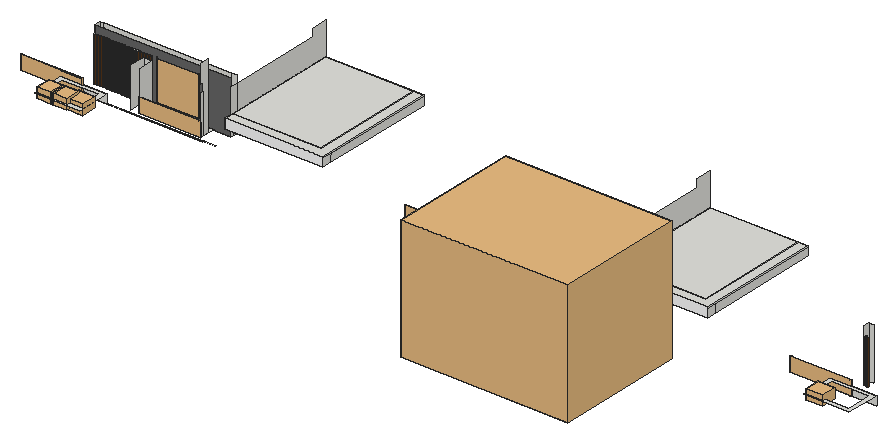
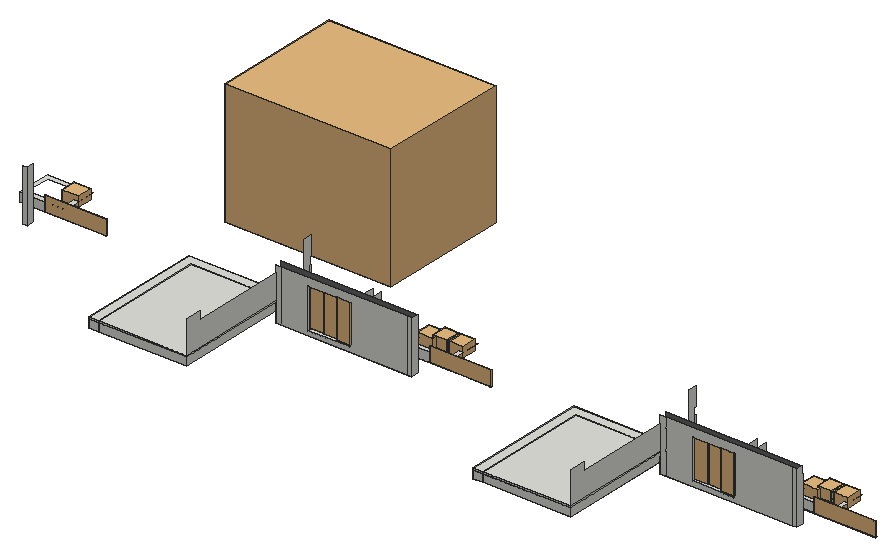
# SketchUp Ruby script. Lengths in inches.
U = 1.inch
M = Sketchup.active_model
def pt(a) = Geom::Point3d.new(a.map { |v| v * U })
def face(e, loops, mat)
  f = e.add_face(loops[0].map { |a| pt(a) })
  loops[1..].each { |l| e.add_face(l.map { |a| pt(a) }).erase! }
  f.material = f.back_material = mat if mat
  f
end
# faces: each face lists its corners as indices into pts; further lists are holes
def faces(e, pts, list, mat = nil) = list.each { |f| face(e, (f[0].is_a?(Array) ? f : [f]).map { |l| l.map { |i| pts[i] } }, mat) }
# xy, xz, yz: faces in a plane at the given z, y or x. An outline is a flat list of corners, or four numbers for a rectangle; further outlines are holes
def ring(l) = l.size == 4 ? [[l[0], l[1]], [l[2], l[1]], [l[2], l[3]], [l[0], l[3]]] : l.each_slice(2).to_a
def flat(e, list, mat, &to3) = list.each { |f| face(e, (f[0].is_a?(Array) ? f : [f]).map { |l| ring(l).map { |u, v| to3.(u, v) } }, mat) }
def xy(e, z, list, mat = nil) = flat(e, list, mat) { |x, y| [x, y, z] }
def xz(e, y, list, mat = nil) = flat(e, list, mat) { |x, z| [x, y, z] }
def yz(e, x, list, mat = nil) = flat(e, list, mat) { |y, z| [x, y, z] }
def lines(e, pts, list) = list.each { |a, b| e.add_line(pt(pts[a]), pt(pts[b])) }
# prism: a flat outline (further loops are holes) pulled along v
def prism(e, loops, v, mat = nil)
  f = face(e, loops, mat); d = Geom::Vector3d.new(v.map { |x| x * U })
  f.pushpull(f.normal.samedirection?(d) ? d.length : -d.length)
end
def box(e, o, s, mat = nil) = prism(e, [[o, [o[0] + s[0], o[1], o[2]], [o[0] + s[0], o[1] + s[1], o[2]], [o[0], o[1] + s[1], o[2]]]], [0, 0, s[2]], mat)
def at(x, y, z, deg = 0) = Geom::Transformation.translation(pt([x, y, z])) * Geom::Transformation.rotation(ORIGIN, Z_AXIS, deg.degrees)
def axes(o, x, y, z) = Geom::Transformation.new([*x, 0, *y, 0, *z, 0, *pt(o).to_a, 1])
def part(name) = M.definitions.add(name)
# library, detail: a bought-in or finely detailed component or shape, given as its bounding box
def library(name, o, s) = part(name).tap { |d| box(d.entities, o, s) }
def detail(e, o, s) = box(e.add_group.entities, o, s)
def put(e, d, t, mat = nil) = e.add_instance(d, t).tap { |i| i.material = mat if mat }
def group(e, t, mat = nil) = e.add_group.tap { |g| g.transformation = t; g.material = mat if mat }.entities
root = M.entities
M.materials.add("Material~3").color = [123, 113, 102]
M.materials.add("[0030_OldLace]").color = [86, 53, 24]
M.materials.add("[0128_White]").color = [255, 255, 255]
M.materials.add("[Slate Light Tile]").color = [104, 104, 104]
M.materials.add("[Wood Veneer 01]").color = [120, 70, 37]
c1 = part("glass-railing")
detail(c1.entities,[0,0,0],[1.26,75.59,33.1875])
c2 = library("Ornamental+Grasses",[-8.33,-8.78,0],[17.11,15.88,10.63])
c3 = library("3DGeom~4_Defintion",[362.52,-15.59,12.6],[288.85,70.11,1000])
c4 = library("3 door",[0,0,0],[74.8,3.9375,43.31])
c5 = library("Sans+titre+(1)+(1)+(2)",[-30.91,-35.46,0],[63.51,67.02,85.79])
xy(root,162.75,[[411.09,845.35,827.91,846.1],[1291.04,845.35,1707.86,846.1],[636.22,888.83,636.22,890.39,634.63,890.39,634.63,888.95,629.22,888.95,629.22,890.39,627.63,890.39,627.63,888.95,622.22,888.95,622.22,890.39,620.63,890.39,620.63,888.95,615.22,888.95,615.22,890.39,613.63,890.39,613.63,888.95,608.22,888.95,608.22,890.39,606.63,890.39,606.63,888.95,601.22,888.95,601.22,890.39,599.63,890.39,599.63,888.95,594.22,888.95,594.22,890.39,592.63,890.39,592.63,888.95,587.22,888.95,587.22,890.39,585.63,890.39,585.63,888.95,580.22,888.95,580.22,890.39,578.63,890.39,578.63,888.95,573.22,888.95,573.22,890.39,571.63,890.39,571.63,888.95,566.22,888.95,566.22,890.39,564.63,890.39,564.63,888.95,559.22,888.95,559.22,890.39,557.63,890.39,557.63,888.95,552.22,888.95,552.22,890.39,550.57,890.39,550.57,888.95,545.16,888.95,545.16,905.7,857.125,905.7,857.125,890.39,676.63,890.39,676.63,888.83,671.22,888.83,671.22,890.39,669.63,890.39,669.63,888.83,664.22,888.83,664.22,890.39,662.63,890.39,662.63,888.83,657.22,888.83,657.22,890.39,655.63,890.39,655.63,888.83,650.22,888.83,650.22,890.39,648.63,890.39,648.63,888.83,643.22,888.83,643.22,890.39,641.63,890.39,641.63,888.83],[1516.16,888.83,1516.16,890.39,1514.58,890.39,1514.58,888.95,1509.16,888.95,1509.16,890.39,1507.58,890.39,1507.58,888.95,1502.16,888.95,1502.16,890.39,1500.58,890.39,1500.58,888.95,1495.16,888.95,1495.16,890.39,1493.58,890.39,1493.58,888.95,1488.16,888.95,1488.16,890.39,1486.58,890.39,1486.58,888.95,1481.16,888.95,1481.16,890.39,1479.58,890.39,1479.58,888.95,1474.16,888.95,1474.16,890.39,1472.58,890.39,1472.58,888.95,1467.16,888.95,1467.16,890.39,1465.58,890.39,1465.58,888.95,1460.16,888.95,1460.16,890.39,1458.58,890.39,1458.58,888.95,1453.16,888.95,1453.16,890.39,1451.58,890.39,1451.58,888.95,1446.16,888.95,1446.16,890.39,1444.58,890.39,1444.58,888.95,1439.16,888.95,1439.16,890.39,1437.58,890.39,1437.58,888.95,1432.16,888.95,1432.16,890.39,1430.52,890.39,1430.52,888.95,1425.1,888.95,1425.1,905.7,1737.07,905.7,1737.07,890.39,1556.58,890.39,1556.58,888.83,1551.16,888.83,1551.16,890.39,1549.58,890.39,1549.58,888.83,1544.16,888.83,1544.16,890.39,1542.58,890.39,1542.58,888.83,1537.16,888.83,1537.16,890.39,1535.58,890.39,1535.58,888.83,1530.16,888.83,1530.16,890.39,1528.58,890.39,1528.58,888.83,1523.16,888.83,1523.16,890.39,1521.58,890.39,1521.58,888.83]])
xy(root,163,[[827.91,845.35,857.125,846.1],[1707.86,845.35,1737.07,846.1]])
xy(root,173.4375,[[687.49,840.97,827.91,877.14],[1567.4375,840.97,1707.86,877.14],[687.6875,890.39,782.75,905.7],[1567.63,890.39,1662.7,905.7]])
xy(root,183.3125,[[[505.35,767.72,609.54,845.35],[514,776.37,600.89,836.7]],[[1385.29,767.72,1489.48,845.35],[1393.94,776.37,1480.84,836.7]],[[2265.24,767.72,2369.43,845.35],[2273.89,776.37,2360.78,836.7]]])
xy(root,186.75,[[1044.04,893.65,1050.1875,895.71],[1052.35,893.65,1058.5,895.71],[1923.98,893.65,1930.13,895.71],[1932.29,893.65,1938.44,895.71],[861.16,894.34,867.3125,895.71],
  [869.48,894.34,875.625,895.71],[877.79,894.34,883.9375,895.71],[886.1,894.34,892.25,895.71],[894.41,894.34,900.5625,895.71],[902.73,894.34,908.875,895.71],
  [911.04,894.34,917.1875,895.71],[919.35,894.34,925.5,895.71],[927.66,894.34,933.8125,895.71],[935.98,894.34,942.125,895.71],[944.29,894.34,950.4375,895.71],
  [952.6,894.34,958.75,895.71],[960.91,894.34,967.0625,895.71],[969.23,894.34,975.375,895.71],[977.54,894.34,983.6875,895.71],[985.85,894.34,992,895.71],
  [994.16,894.34,1000.3125,895.71],[1002.48,894.34,1008.625,895.71],[1010.79,894.34,1016.9375,895.71],[1019.1,894.34,1025.25,895.71],[1027.41,894.34,1033.5625,895.71],
  [1035.73,894.34,1041.875,895.71],[1741.11,894.34,1747.26,895.71],[1749.42,894.34,1755.57,895.71],[1757.73,894.34,1763.88,895.71],[1766.04,894.34,1772.19,895.71],
  [1774.36,894.34,1780.51,895.71],[1782.67,894.34,1788.82,895.71],[1790.98,894.34,1797.13,895.71],[1799.29,894.34,1805.44,895.71],[1807.61,894.34,1813.76,895.71],
  [1815.92,894.34,1822.07,895.71],[1824.23,894.34,1830.38,895.71],[1832.54,894.34,1838.69,895.71],[1840.86,894.34,1847.01,895.71],[1849.17,894.34,1855.32,895.71],
  [1857.48,894.34,1863.63,895.71],[1865.79,894.34,1871.94,895.71],[1874.11,894.34,1880.26,895.71],[1882.42,894.34,1888.57,895.71],[1890.73,894.34,1896.88,895.71],
  [1899.04,894.34,1905.19,895.71],[1907.36,894.34,1913.51,895.71],[1915.67,894.34,1921.82,895.71],[[857.125,895.71,1058.5,1160.85],[865.59,904.18,1047.28,1152.375]],[[1737.07,895.71,1938.44,1160.85],[1745.54,904.18,1927.22,1152.375]]])
xy(root,186.75,[[857.125,873.28,857.125,895.71,861.16,895.71,861.16,894.34,867.3125,894.34,867.3125,895.71,869.48,895.71,869.48,894.34,875.625,894.34,875.625,895.71,877.79,895.71,877.79,894.34,883.9375,894.34,883.9375,895.71,886.1,895.71,886.1,894.34,892.25,894.34,892.25,895.71,894.41,895.71,894.41,894.34,900.5625,894.34,900.5625,895.71,902.73,895.71,902.73,894.34,908.875,894.34,908.875,895.71,911.04,895.71,911.04,894.34,917.1875,894.34,917.1875,895.71,919.35,895.71,919.35,894.34,925.5,894.34,925.5,895.71,927.66,895.71,927.66,894.34,933.8125,894.34,933.8125,895.71,935.98,895.71,935.98,894.34,942.125,894.34,942.125,895.71,944.29,895.71,944.29,894.34,950.4375,894.34,950.4375,895.71,952.6,895.71,952.6,894.34,958.75,894.34,958.75,895.71,960.91,895.71,960.91,894.34,967.0625,894.34,967.0625,895.71,969.23,895.71,969.23,894.34,975.375,894.34,975.375,895.71,977.54,895.71,977.54,894.34,983.6875,894.34,983.6875,895.71,985.85,895.71,985.85,894.34,992,894.34,992,895.71,994.16,895.71,994.16,894.34,1000.3125,894.34,1000.3125,895.71,1002.48,895.71,1002.48,894.34,1008.625,894.34,1008.625,895.71,1010.79,895.71,1010.79,894.34,1016.9375,894.34,1016.9375,895.71,1019.1,895.71,1019.1,894.34,1025.25,894.34,1025.25,895.71,1027.41,895.71,1027.41,894.34,1033.5625,894.34,1033.5625,895.71,1035.73,895.71,1035.73,894.34,1041.875,894.34,1041.875,895.71,1044.04,895.71,1044.04,893.65,1050.1875,893.65,1050.1875,895.71,1052.35,895.71,1052.35,893.65,1058.5,893.65,1058.5,895.71,1080.92,895.71,1080.92,873.28],[1737.07,873.28,1737.07,895.71,1741.11,895.71,1741.11,894.34,1747.26,894.34,1747.26,895.71,1749.42,895.71,1749.42,894.34,1755.57,894.34,1755.57,895.71,1757.73,895.71,1757.73,894.34,1763.88,894.34,1763.88,895.71,1766.04,895.71,1766.04,894.34,1772.19,894.34,1772.19,895.71,1774.36,895.71,1774.36,894.34,1780.51,894.34,1780.51,895.71,1782.67,895.71,1782.67,894.34,1788.82,894.34,1788.82,895.71,1790.98,895.71,1790.98,894.34,1797.13,894.34,1797.13,895.71,1799.29,895.71,1799.29,894.34,1805.44,894.34,1805.44,895.71,1807.61,895.71,1807.61,894.34,1813.76,894.34,1813.76,895.71,1815.92,895.71,1815.92,894.34,1822.07,894.34,1822.07,895.71,1824.23,895.71,1824.23,894.34,1830.38,894.34,1830.38,895.71,1832.54,895.71,1832.54,894.34,1838.69,894.34,1838.69,895.71,1840.86,895.71,1840.86,894.34,1847.01,894.34,1847.01,895.71,1849.17,895.71,1849.17,894.34,1855.32,894.34,1855.32,895.71,1857.48,895.71,1857.48,894.34,1863.63,894.34,1863.63,895.71,1865.79,895.71,1865.79,894.34,1871.94,894.34,1871.94,895.71,1874.11,895.71,1874.11,894.34,1880.26,894.34,1880.26,895.71,1882.42,895.71,1882.42,894.34,1888.57,894.34,1888.57,895.71,1890.73,895.71,1890.73,894.34,1896.88,894.34,1896.88,895.71,1899.04,895.71,1899.04,894.34,1905.19,894.34,1905.19,895.71,1907.36,895.71,1907.36,894.34,1913.51,894.34,1913.51,895.71,1915.67,895.71,1915.67,894.34,1921.82,894.34,1921.82,895.71,1923.98,895.71,1923.98,893.65,1930.13,893.65,1930.13,895.71,1932.29,895.71,1932.29,893.65,1938.44,893.65,1938.44,895.71,1960.87,895.71,1960.87,873.28],[1058.5,895.71,1080.92,1160.85],[1938.44,895.71,1960.87,1160.85]],"[Wood Veneer 01]")
xy(root,204.8125,[[[857.125,895.71,1058.5,1160.85],[865.59,904.18,1047.28,1152.375]],[1058.5,895.71,1080.92,1160.85],[[1737.07,895.71,1938.44,1160.85],[1745.54,904.18,1927.22,1152.375]],[1938.44,895.71,1960.87,1160.85]])
xy(root,208.375,[[857.125,873.28,1080.92,873.28,1080.92,1160.85,1058.5,1160.85,1058.5,895.71,857.125,895.71],[1737.07,873.28,1960.87,873.28,1960.87,1160.85,1938.44,1160.85,1938.44,895.71,1737.07,895.71],[857.125,895.71,1058.5,1160.85],[1737.07,895.71,1938.44,1160.85]])
xz(root,845.35,[[505.35,162.75,609.54,183.3125],[1385.29,162.75,1489.48,183.3125],[2265.24,162.75,2369.43,183.3125]])
xz(root,873.28,[[857.125,186.75,1080.92,208.375],[1737.07,186.75,1960.87,208.375]],"[0128_White]")
xz(root,877.14,[[667.84,173.4375,687.49,264.75],[1547.79,173.4375,1567.4375,264.75]])
xz(root,888.83,[[636.22,162.75,641.63,264.75],[643.22,162.75,648.63,264.75],[650.22,162.75,655.63,264.75],[657.22,162.75,662.63,264.75],[664.22,162.75,669.63,264.75],
  [671.22,162.75,676.63,264.75],[1516.16,162.75,1521.58,264.75],[1523.16,162.75,1528.58,264.75],[1530.16,162.75,1535.58,264.75],[1537.16,162.75,1542.58,264.75],
  [1544.16,162.75,1549.58,264.75],[1551.16,162.75,1556.58,264.75]],"[0030_OldLace]")
xz(root,888.95,[[545.16,162.75,550.57,264.75],[552.22,162.75,557.63,264.75],[559.22,162.75,564.63,264.75],[566.22,162.75,571.63,264.75],[573.22,162.75,578.63,264.75],
  [580.22,162.75,585.63,264.75],[587.22,162.75,592.63,264.75],[594.22,162.75,599.63,264.75],[601.22,162.75,606.63,264.75],[608.22,162.75,613.63,264.75],
  [615.22,162.75,620.63,264.75],[622.22,162.75,627.63,264.75],[629.22,162.75,634.63,264.75],[1425.1,162.75,1430.52,264.75],[1432.16,162.75,1437.58,264.75],
  [1439.16,162.75,1444.58,264.75],[1446.16,162.75,1451.58,264.75],[1453.16,162.75,1458.58,264.75],[1460.16,162.75,1465.58,264.75],[1467.16,162.75,1472.58,264.75],
  [1474.16,162.75,1479.58,264.75],[1481.16,162.75,1486.58,264.75],[1488.16,162.75,1493.58,264.75],[1495.16,162.75,1500.58,264.75],[1502.16,162.75,1507.58,264.75],
  [1509.16,162.75,1514.58,264.75],[2305.05,162.75,2310.46,264.75],[2312.11,162.75,2317.52,264.75]],"[0030_OldLace]")
xz(root,890.39,[[[550.57,162.75,552.22,162.75,552.22,264.75,557.63,264.75,557.63,162.75,559.22,162.75,559.22,264.75,564.63,264.75,564.63,162.75,566.22,162.75,566.22,264.75,571.63,264.75,571.63,162.75,573.22,162.75,573.22,264.75,578.63,264.75,578.63,162.75,580.22,162.75,580.22,264.75,585.63,264.75,585.63,162.75,587.22,162.75,587.22,264.75,592.63,264.75,592.63,162.75,594.22,162.75,594.22,264.75,599.63,264.75,599.63,162.75,601.22,162.75,601.22,264.75,606.63,264.75,606.63,162.75,608.22,162.75,608.22,264.75,613.63,264.75,613.63,162.75,615.22,162.75,615.22,264.75,620.63,264.75,620.63,162.75,622.22,162.75,622.22,264.75,627.63,264.75,627.63,162.75,629.22,162.75,629.22,264.75,634.63,264.75,634.63,162.75,636.22,162.75,636.22,264.75,641.63,264.75,641.63,162.75,643.22,162.75,643.22,264.75,648.63,264.75,648.63,162.75,650.22,162.75,650.22,264.75,655.63,264.75,655.63,162.75,657.22,162.75,657.22,264.75,662.63,264.75,662.63,162.75,664.22,162.75,664.22,264.75,669.63,264.75,669.63,162.75,671.22,162.75,671.22,264.75,676.63,264.75,676.63,162.75,857.125,162.75,857.125,282.75,545.16,282.75,545.16,264.75,550.57,264.75],[687.6875,173.4375,782.75,264.75]],[[1430.52,162.75,1432.16,162.75,1432.16,264.75,1437.58,264.75,1437.58,162.75,1439.16,162.75,1439.16,264.75,1444.58,264.75,1444.58,162.75,1446.16,162.75,1446.16,264.75,1451.58,264.75,1451.58,162.75,1453.16,162.75,1453.16,264.75,1458.58,264.75,1458.58,162.75,1460.16,162.75,1460.16,264.75,1465.58,264.75,1465.58,162.75,1467.16,162.75,1467.16,264.75,1472.58,264.75,1472.58,162.75,1474.16,162.75,1474.16,264.75,1479.58,264.75,1479.58,162.75,1481.16,162.75,1481.16,264.75,1486.58,264.75,1486.58,162.75,1488.16,162.75,1488.16,264.75,1493.58,264.75,1493.58,162.75,1495.16,162.75,1495.16,264.75,1500.58,264.75,1500.58,162.75,1502.16,162.75,1502.16,264.75,1507.58,264.75,1507.58,162.75,1509.16,162.75,1509.16,264.75,1514.58,264.75,1514.58,162.75,1516.16,162.75,1516.16,264.75,1521.58,264.75,1521.58,162.75,1523.16,162.75,1523.16,264.75,1528.58,264.75,1528.58,162.75,1530.16,162.75,1530.16,264.75,1535.58,264.75,1535.58,162.75,1537.16,162.75,1537.16,264.75,1542.58,264.75,1542.58,162.75,1544.16,162.75,1544.16,264.75,1549.58,264.75,1549.58,162.75,1551.16,162.75,1551.16,264.75,1556.58,264.75,1556.58,162.75,1737.07,162.75,1737.07,282.75,1425.1,282.75,1425.1,264.75,1430.52,264.75],[1567.63,173.4375,1662.7,264.75]]],"[Slate Light Tile]")
xz(root,895.71,[[857.125,186.75,1058.5,204.8125],[1058.5,186.75,1080.92,204.8125],[1737.07,186.75,1938.44,204.8125],[1938.44,186.75,1960.87,204.8125],[857.125,204.8125,1058.5,208.375],
  [1737.07,204.8125,1938.44,208.375]])
xz(root,904.18,[[865.59,186.75,1047.28,204.8125],[1745.54,186.75,1927.22,204.8125]])
xz(root,905.7,[[545.16,162.75,554.54,282.75],[[554.54,162.75,844.86,282.75],[687.6875,173.4375,782.75,264.75]],[844.86,162.75,857.125,282.75],[1425.1,162.75,1434.48,282.75],[[1434.48,162.75,1724.81,282.75],[1567.63,173.4375,1662.7,264.75]],
  [1724.81,162.75,1737.07,282.75],[2305.05,162.75,2314.43,282.75]])
xz(root,1152.375,[[865.59,186.75,1047.28,204.8125],[1745.54,186.75,1927.22,204.8125]])
xz(root,1160.85,[[857.125,186.75,1058.5,204.8125],[1058.5,186.75,1080.92,204.8125],[1737.07,186.75,1938.44,204.8125],[1938.44,186.75,1960.87,204.8125],[857.125,204.8125,1058.5,208.375],
  [1058.5,204.8125,1080.92,208.375],[1737.07,204.8125,1938.44,208.375],[1938.44,204.8125,1960.87,208.375]])
yz(root,545.16,[[888.95,162.75,888.95,264.75,890.39,264.75,890.39,282.75,905.7,282.75,905.7,162.75]])
yz(root,550.57,[[888.95,162.75,890.39,264.75]])
yz(root,552.22,[[888.95,162.75,890.39,264.75]])
yz(root,557.63,[[888.95,162.75,890.39,264.75]])
yz(root,559.22,[[888.95,162.75,890.39,264.75]])
yz(root,564.63,[[888.95,162.75,890.39,264.75]])
yz(root,566.22,[[888.95,162.75,890.39,264.75]])
yz(root,571.63,[[888.95,162.75,890.39,264.75]])
yz(root,573.22,[[888.95,162.75,890.39,264.75]])
yz(root,578.63,[[888.95,162.75,890.39,264.75]])
yz(root,580.22,[[888.95,162.75,890.39,264.75]])
yz(root,585.63,[[888.95,162.75,890.39,264.75]])
yz(root,587.22,[[888.95,162.75,890.39,264.75]])
yz(root,592.63,[[888.95,162.75,890.39,264.75]])
yz(root,594.22,[[888.95,162.75,890.39,264.75]])
yz(root,599.63,[[888.95,162.75,890.39,264.75]])
yz(root,601.22,[[888.95,162.75,890.39,264.75]])
yz(root,606.63,[[888.95,162.75,890.39,264.75]])
yz(root,608.22,[[888.95,162.75,890.39,264.75]])
yz(root,613.63,[[888.95,162.75,890.39,264.75]])
yz(root,615.22,[[888.95,162.75,890.39,264.75]])
yz(root,620.63,[[888.95,162.75,890.39,264.75]])
yz(root,622.22,[[888.95,162.75,890.39,264.75]])
yz(root,627.63,[[888.95,162.75,890.39,264.75]])
yz(root,629.22,[[888.95,162.75,890.39,264.75]])
yz(root,634.63,[[888.95,162.75,890.39,264.75]])
yz(root,636.22,[[888.83,162.75,890.39,264.75]])
yz(root,641.63,[[888.83,162.75,890.39,264.75]])
yz(root,643.22,[[888.83,162.75,890.39,264.75]])
yz(root,648.63,[[888.83,162.75,890.39,264.75]])
yz(root,650.22,[[888.83,162.75,890.39,264.75]],"[0030_OldLace]")
yz(root,655.63,[[888.83,162.75,890.39,264.75]])
yz(root,657.22,[[888.83,162.75,890.39,264.75]],"[0030_OldLace]")
yz(root,662.63,[[888.83,162.75,890.39,264.75]])
yz(root,664.22,[[888.83,162.75,890.39,264.75]],"[0030_OldLace]")
yz(root,667.84,[[840.97,173.4375,877.14,264.75]])
yz(root,669.63,[[888.83,162.75,890.39,264.75]])
yz(root,671.22,[[888.83,162.75,890.39,264.75]],"[0030_OldLace]")
yz(root,676.63,[[888.83,162.75,890.39,264.75]])
yz(root,687.49,[[840.97,173.4375,877.14,264.75]])
yz(root,687.6875,[[890.39,173.4375,905.7,264.75]])
yz(root,782.75,[[890.39,173.4375,905.7,264.75]])
yz(root,827.91,[[845.35,162.75,846.1,163],[840.97,173.4375,846.1,264.75],[846.1,173.4375,846.1,264.75,845.35,264.75,845.35,282.75,840.97,282.75,840.97,324.5625,861.24,324.5625,861.24,173.4375]])
yz(root,857.125,[[890.39,162.75,895.71,186.75],[895.71,162.75,905.7,186.75],[873.28,186.75,890.39,204.8125],[890.39,186.75,895.71,204.8125],[895.71,186.75,905.7,204.8125],
  [905.7,186.75,1160.85,204.8125],[873.28,204.8125,890.39,208.375],[890.39,204.8125,895.71,208.375],[895.71,204.8125,905.7,208.375],[905.7,204.8125,1160.85,208.375],
  [890.39,208.375,905.7,264.75],[905.7,208.375,1160.85,208.375,1160.85,282.75,1122.97,282.75,1122.97,264.75,905.7,264.75]])
yz(root,865.59,[[904.18,186.75,905.7,204.8125],[905.7,186.75,1152.375,204.8125]])
yz(root,1047.28,[[904.18,186.75,1152.375,204.8125]])
yz(root,1058.5,[[895.71,186.75,1160.85,204.8125],[895.71,204.8125,1160.85,208.375]])
yz(root,1080.92,[[873.28,186.75,895.71,204.8125],[895.71,186.75,1160.85,204.8125],[873.28,204.8125,1160.85,208.375]])
yz(root,1425.1,[[888.95,162.75,888.95,264.75,890.39,264.75,890.39,282.75,905.7,282.75,905.7,162.75]])
yz(root,1430.52,[[888.95,162.75,890.39,264.75]])
yz(root,1432.16,[[888.95,162.75,890.39,264.75]])
yz(root,1437.58,[[888.95,162.75,890.39,264.75]])
yz(root,1439.16,[[888.95,162.75,890.39,264.75]])
yz(root,1444.58,[[888.95,162.75,890.39,264.75]])
yz(root,1446.16,[[888.95,162.75,890.39,264.75]])
yz(root,1451.58,[[888.95,162.75,890.39,264.75]])
yz(root,1453.16,[[888.95,162.75,890.39,264.75]])
yz(root,1458.58,[[888.95,162.75,890.39,264.75]])
yz(root,1460.16,[[888.95,162.75,890.39,264.75]])
yz(root,1465.58,[[888.95,162.75,890.39,264.75]])
yz(root,1467.16,[[888.95,162.75,890.39,264.75]])
yz(root,1472.58,[[888.95,162.75,890.39,264.75]])
yz(root,1474.16,[[888.95,162.75,890.39,264.75]])
yz(root,1479.58,[[888.95,162.75,890.39,264.75]])
yz(root,1481.16,[[888.95,162.75,890.39,264.75]])
yz(root,1486.58,[[888.95,162.75,890.39,264.75]])
yz(root,1488.16,[[888.95,162.75,890.39,264.75]])
yz(root,1493.58,[[888.95,162.75,890.39,264.75]])
yz(root,1495.16,[[888.95,162.75,890.39,264.75]])
yz(root,1500.58,[[888.95,162.75,890.39,264.75]])
yz(root,1502.16,[[888.95,162.75,890.39,264.75]])
yz(root,1507.58,[[888.95,162.75,890.39,264.75]])
yz(root,1509.16,[[888.95,162.75,890.39,264.75]])
yz(root,1514.58,[[888.95,162.75,890.39,264.75]])
yz(root,1516.16,[[888.83,162.75,890.39,264.75]])
yz(root,1521.58,[[888.83,162.75,890.39,264.75]])
yz(root,1523.16,[[888.83,162.75,890.39,264.75]])
yz(root,1528.58,[[888.83,162.75,890.39,264.75]])
yz(root,1530.16,[[888.83,162.75,890.39,264.75]],"[0030_OldLace]")
yz(root,1535.58,[[888.83,162.75,890.39,264.75]])
yz(root,1537.16,[[888.83,162.75,890.39,264.75]],"[0030_OldLace]")
yz(root,1542.58,[[888.83,162.75,890.39,264.75]])
yz(root,1544.16,[[888.83,162.75,890.39,264.75]],"[0030_OldLace]")
yz(root,1547.79,[[840.97,173.4375,877.14,264.75]])
yz(root,1549.58,[[888.83,162.75,890.39,264.75]])
yz(root,1551.16,[[888.83,162.75,890.39,264.75]],"[0030_OldLace]")
yz(root,1556.58,[[888.83,162.75,890.39,264.75]])
yz(root,1567.4375,[[840.97,173.4375,877.14,264.75]])
yz(root,1567.63,[[890.39,173.4375,905.7,264.75]])
yz(root,1662.7,[[890.39,173.4375,905.7,264.75]])
yz(root,1707.86,[[845.35,162.75,846.1,163],[840.97,173.4375,846.1,264.75],[846.1,173.4375,846.1,264.75,845.35,264.75,845.35,282.75,840.97,282.75,840.97,324.5625,861.24,324.5625,861.24,173.4375]])
yz(root,1737.07,[[890.39,162.75,895.71,186.75],[895.71,162.75,905.7,186.75],[873.28,186.75,890.39,204.8125],[890.39,186.75,895.71,204.8125],[895.71,186.75,905.7,204.8125],
  [905.7,186.75,1160.85,204.8125],[873.28,204.8125,890.39,208.375],[890.39,204.8125,895.71,208.375],[895.71,204.8125,905.7,208.375],[905.7,204.8125,1160.85,208.375],
  [890.39,208.375,905.7,264.75],[905.7,208.375,1160.85,208.375,1160.85,282.75,1122.97,282.75,1122.97,264.75,905.7,264.75]])
yz(root,1745.54,[[904.18,186.75,905.7,204.8125],[905.7,186.75,1152.375,204.8125]])
yz(root,1927.22,[[904.18,186.75,1152.375,204.8125]])
yz(root,1938.44,[[895.71,186.75,1160.85,204.8125],[895.71,204.8125,1160.85,208.375]])
yz(root,1960.87,[[873.28,186.75,895.71,204.8125],[895.71,186.75,1160.85,204.8125],[873.28,204.8125,1160.85,208.375]])
yz(root,2305.05,[[888.95,162.75,888.95,264.75,890.39,264.75,890.39,282.75,905.7,282.75,905.7,162.75]])
yz(root,2310.46,[[888.95,162.75,890.39,264.75]])
yz(root,2312.11,[[888.95,162.75,890.39,264.75]])
p = [[679.79,890.39,264.75],[679.79,890.39,162.75],[1559.74,890.39,264.75],[1559.74,890.39,162.75]]
lines(root,p,[[0,1],[2,3]])
put(root,c1,axes([412.04,845.7,162.75],[0,-1,0],[1.87,0,0],[0,0,1]))
put(root,c2,axes([525.51,791.57,170.63],[2.19,0,0],[0,2.19,0],[0,0,2.19]))
put(root,c2,axes([557.32,791.57,170.63],[2.19,0,0],[0,2.19,0],[0,0,2.19]))
put(root,c2,axes([588.47,798.1875,167.75],[2.19,0,0],[0,2.19,0],[0,0,2.19]))
put(root,c3,axes([645.83,905.3125,176.31],[0.11056,0,0],[0,-0.05859,0],[0,0,0.08734]),"Material~3")
put(root,c3,axes([677.43,901.24,176.31],[0.11056,0,0],[0,-0.05859,0],[0,0,0.08734]),"Material~3")
put(root,c4,axes([687.6875,890.39,173.4375],[1.27084,0,0],[0,1.38,0],[0,0,2.15904]))
put(root,c1,axes([687.43,841,173.4375],[0,-1,0],[1.86,0,0],[0,0,1]))
put(root,c3,axes([710.74,901.24,176.31],[0.11056,0,0],[0,-0.05859,0],[0,0,0.08734]),"Material~3")
put(root,c1,axes([1291.98,845.7,162.75],[0,-1,0],[1.87,0,0],[0,0,1]))
put(root,c2,axes([1405.45,791.57,170.63],[2.19,0,0],[0,2.19,0],[0,0,2.19]))
put(root,c2,axes([1437.26,791.57,170.63],[2.19,0,0],[0,2.19,0],[0,0,2.19]))
put(root,c2,axes([1468.42,798.1875,167.75],[2.19,0,0],[0,2.19,0],[0,0,2.19]))
put(root,c3,axes([1525.77,905.3125,176.31],[0.11056,0,0],[0,-0.05859,0],[0,0,0.08734]),"Material~3")
put(root,c3,axes([1557.37,901.24,176.31],[0.11056,0,0],[0,-0.05859,0],[0,0,0.08734]),"Material~3")
put(root,c4,axes([1567.63,890.39,173.4375],[1.27084,0,0],[0,1.38,0],[0,0,2.15904]))
put(root,c1,axes([1567.38,841,173.4375],[0,-1,0],[1.86,0,0],[0,0,1]))
put(root,c3,axes([1590.68,901.24,176.31],[0.11056,0,0],[0,-0.05859,0],[0,0,0.08734]),"Material~3")
put(root,c5,axes([1627.32,572.03,335.18],[0,0,-4.44],[0,4.44,0],[4.44,0,0]))
put(root,c1,axes([2171.93,845.7,162.75],[0,-1,0],[1.87,0,0],[0,0,1]))
put(root,c2,axes([2285.39,791.57,170.63],[2.19,0,0],[0,2.19,0],[0,0,2.19]))
